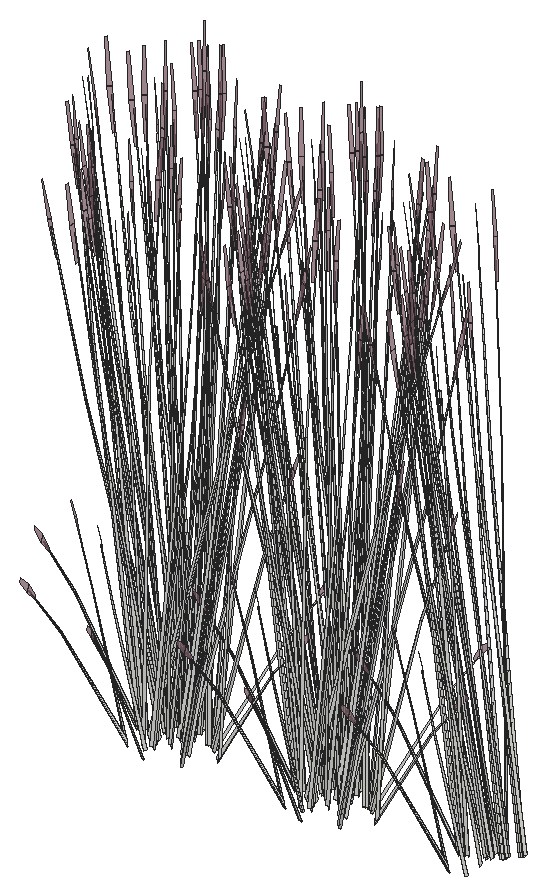
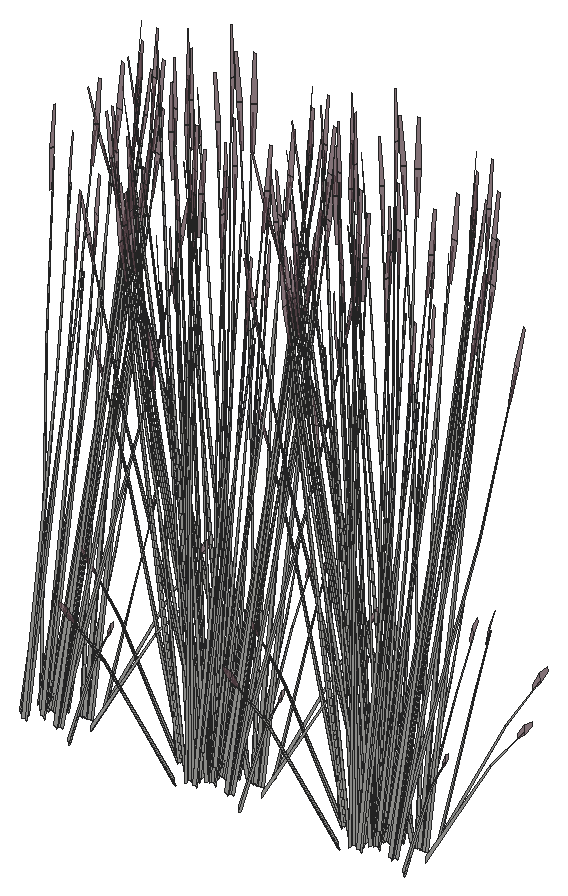
# SketchUp Ruby script. Lengths in inches.
U = 1.inch
M = Sketchup.active_model
def pt(a) = Geom::Point3d.new(a.map { |v| v * U })
def face(e, loops, mat)
  f = e.add_face(loops[0].map { |a| pt(a) })
  loops[1..].each { |l| e.add_face(l.map { |a| pt(a) }).erase! }
  f.material = f.back_material = mat if mat
  f
end
# faces: each face lists its corners as indices into pts; further lists are holes
def faces(e, pts, list, mat = nil) = list.each { |f| face(e, (f[0].is_a?(Array) ? f : [f]).map { |l| l.map { |i| pts[i] } }, mat) }
# xy, xz, yz: faces in a plane at the given z, y or x. An outline is a flat list of corners, or four numbers for a rectangle; further outlines are holes
def ring(l) = l.size == 4 ? [[l[0], l[1]], [l[2], l[1]], [l[2], l[3]], [l[0], l[3]]] : l.each_slice(2).to_a
def flat(e, list, mat, &to3) = list.each { |f| face(e, (f[0].is_a?(Array) ? f : [f]).map { |l| ring(l).map { |u, v| to3.(u, v) } }, mat) }
def xy(e, z, list, mat = nil) = flat(e, list, mat) { |x, y| [x, y, z] }
def xz(e, y, list, mat = nil) = flat(e, list, mat) { |x, z| [x, y, z] }
def yz(e, x, list, mat = nil) = flat(e, list, mat) { |y, z| [x, y, z] }
def lines(e, pts, list) = list.each { |a, b| e.add_line(pt(pts[a]), pt(pts[b])) }
# prism: a flat outline (further loops are holes) pulled along v
def prism(e, loops, v, mat = nil)
  f = face(e, loops, mat); d = Geom::Vector3d.new(v.map { |x| x * U })
  f.pushpull(f.normal.samedirection?(d) ? d.length : -d.length)
end
def box(e, o, s, mat = nil) = prism(e, [[o, [o[0] + s[0], o[1], o[2]], [o[0] + s[0], o[1] + s[1], o[2]], [o[0], o[1] + s[1], o[2]]]], [0, 0, s[2]], mat)
def at(x, y, z, deg = 0) = Geom::Transformation.translation(pt([x, y, z])) * Geom::Transformation.rotation(ORIGIN, Z_AXIS, deg.degrees)
def axes(o, x, y, z) = Geom::Transformation.new([*x, 0, *y, 0, *z, 0, *pt(o).to_a, 1])
def part(name) = M.definitions.add(name)
# library, detail: a bought-in or finely detailed component or shape, given as its bounding box
def library(name, o, s) = part(name).tap { |d| box(d.entities, o, s) }
def detail(e, o, s) = box(e.add_group.entities, o, s)
def put(e, d, t, mat = nil) = e.add_instance(d, t).tap { |i| i.material = mat if mat }
def group(e, t, mat = nil) = e.add_group.tap { |g| g.transformation = t; g.material = mat if mat }.entities
root = M.entities
M.materials.add("LightPink_Translucent").color = [144, 107, 117]
M.materials["LightPink_Translucent"].alpha = 0.75
c1 = part("blade")
p = [[2.15,0.21,22],[0,0.17,0],[0.09,0.45,0],[2.18,0.31,22],[2.29,0.31,22],[0.38,0.45,0],
  [2.48,0.24,33],[2.49,0.24,33],[2.48,0.22,33]]
faces(c1.entities,p,[[0,1,2,3],[4,5,2,3],[6,3,4,7],[8,0,3,6]])
c2 = part("seeds")
p = [[0.3,-0.1,1.38],[-0.01,-0.03,1.59],[-0.01,-0.03,0.03],[0.14,-0.07,-0.07],[0.29,-0.03,3],[0.15,0.01,3.11]]
faces(c2.entities,p,[[0,1,2,3],[1,0,4,5]],"LightPink_Translucent")
c3 = part("blade with seeds")
put(c3.entities,c1,at(0,0,0))
put(c3.entities,c2,axes([2.4,0.25,30.99],[1.5799,-0.05474,1.17369],[-0.12525,1.92788,0.29478],[-0.07173,-0.02425,1.56792]))
put(root,c3,axes([242.16,53.45,256.49],[0.01927,0.0963,1.76342],[-0.38846,0.5029,-0.26939],[-0.27592,-0.02535,0.30037]))
put(root,c3,axes([241.95,56.15,256.49],[0.10192,0.06105,1.76342],[0.17281,0.56562,-0.26939],[-0.22588,0.12062,0.30037]))
put(root,c3,axes([244.7,54.32,257.06],[-0.79037,-0.10018,-0.62353],[0.16679,-0.61794,-0.16365],[-0.23587,-0.07488,1.37633]))
put(root,c3,axes([243.66,55.49,257.02],[-0.7111,-0.30552,-0.49651],[0.42504,-0.54784,0],[-0.16196,-0.06958,1.57504]))
put(root,c3,axes([243.35,50.94,256.49],[-0.0736,0.08049,1.76342],[-0.74378,0.17355,-0.26939],[-0.17968,-0.15788,0.30037]))
put(root,c3,axes([244.1,55.86,257.375],[-0.47504,0.61229,0],[-0.79476,-0.34146,-0.51607],[-0.18101,-0.07777,1.63711]))
put(root,c3,axes([242.89,51.25,257.13],[-0.21918,0.49894,-0.03893],[-0.6746,-0.15348,-0.17649],[-0.10242,-0.08161,0.58215]))
put(root,c3,axes([245.6,54.42,257.67],[-0.76714,0.40567,-0.29095],[-0.51013,-0.57321,-0.50002],[-0.18927,-0.05821,1.59708]))
put(root,c3,axes([242.53,53.53,257.375],[-0.95008,0,0],[0,-0.68292,-0.51607],[0,-0.15554,1.63711]))
put(root,c3,axes([243.86,55.27,257.03],[-0.17848,-0.53243,-0.30978],[0.70886,-0.15119,0.30978],[-0.1429,-0.0614,1.38974]))
put(root,c3,axes([246.11,54.86,257.06],[-0.51177,0.45928,-0.62353],[-0.63575,-0.41646,-0.16365],[-0.20507,0.11457,1.37633]))
put(root,c3,axes([243.26,53.35,257.33],[-0.70674,0.51372,0.30756],[-0.70717,-0.50832,-0.36492],[-0.02468,-0.14589,1.64885]))
put(root,c3,axes([246.46,54.6,257.46],[-0.74193,-0.49181,-0.25192],[0.6243,-0.55226,0.5513],[-0.19979,0.05753,1.68216]))
put(root,c3,axes([245.11,54.13,257.21],[-0.45644,-0.51287,-0.44739],[0.69137,-0.36116,0.21531],[-0.14771,-0.06346,1.43643]))
put(root,c3,axes([246.08,54.5,257.21],[-0.82508,0.03772,-0.44739],[-0.07462,-0.62614,0.21531],[-0.14771,0.06346,1.43643]))
put(root,c3,axes([245.18,54.42,257.4375],[0.20138,-0.72405,-0.23429],[0.95485,0.12621,0.51271],[-0.16685,-0.09999,1.5644]))
put(root,c3,axes([246.95,56.11,257.02],[-0.7111,0.30552,-0.49651],[-0.42504,-0.54784,0],[-0.16196,0.06958,1.57504]))
put(root,c3,axes([242.74,53.07,257.02],[0,-0.61104,-0.49651],[0.85008,0,0],[0,-0.13917,1.57504]))
put(root,c3,axes([247,55.95,257.19],[-0.46912,-0.61443,-0.05142],[0.79476,-0.34146,0.51607],[-0.19584,0.0585,1.6363]))
put(root,c3,axes([246.78,55.87,257.03],[-0.70886,-0.15119,-0.30978],[0.17848,-0.53243,0.30978],[-0.1429,0.0614,1.38974]))
put(root,c3,axes([244.96,53.77,257.67],[-0.85568,-0.29155,-0.29095],[0.41201,-0.61537,-0.50002],[-0.02689,-0.15109,1.59708]))
put(root,c3,axes([246.66,54.33,257.67],[0.08854,0.69723,-0.29095],[-0.92215,0.04216,-0.50002],[-0.16238,0.09287,1.59708]))
put(root,c3,axes([244.58,53.15,257.1],[-0.31203,-0.62659,-0.69835],[0.89884,-0.22566,-0.18329],[-0.03449,-0.21218,1.54149]))
put(root,c3,axes([243.1,53.08,257.03],[0.53038,-0.38124,-0.30978],[0.53038,0.38124,0.30978],[0,-0.1228,1.38974]))
put(root,c3,axes([245.5,50.62,257.13],[-0.52505,0.35054,-0.03893],[-0.48109,-0.38392,-0.17649],[-0.03387,-0.10878,0.58215]))
put(root,c3,axes([245.82,55.33,257.2],[-0.76598,-0.27433,0],[0.36864,-0.57001,0],[0,0,1.62707]))
put(root,c3,axes([247.6,56.02,257.375],[0.47504,0.61229,0],[-0.79476,0.34146,-0.51607],[-0.18101,0.07777,1.63711]))
put(root,c3,axes([246.63,54.01,257.3],[-0.70674,-0.52593,-0.06131],[0.70717,-0.52625,0],[-0.02468,-0.01837,1.75571]))
put(root,c3,axes([247.02,55.63,257.33],[0.95122,0.19861,0.30756],[-0.23797,0.7099,-0.36492],[-0.15744,0.08885,1.64885]))
put(root,c3,axes([245.63,50.1875,256.49],[-0.12744,0.02202,1.76342],[-0.70477,-0.24781,-0.26939],[0.01183,-0.2067,0.30037]))
put(root,c3,axes([245.05,53.32,257.21],[0.36864,-0.55059,-0.44739],[0.76598,0.26498,0.21531],[0,-0.12692,1.43643]))
put(root,c3,axes([246,55.09,257.2],[-0.24791,-0.5268,0],[0.70791,-0.18448,0],[0,0,1.54371]))
put(root,c3,axes([247,54.05,257.21],[-0.36864,0.55059,-0.44739],[-0.76598,-0.26498,0.21531],[0,0.12692,1.43643]))
put(root,c3,axes([246.39,53.46,257.21],[0,-0.70701,0],[0.95008,0,0],[0,0,1.79456]))
put(root,c3,axes([246.87,53.74,257.29],[0,0.70667,-0.05637],[-0.95008,0,0],[0,0.02221,1.79368]))
put(root,c3,axes([246.42,55.11,257.29],[0.33034,0.70197,-0.06012],[-0.94388,0.24598,0],[0.01154,0.02451,1.72173]))
put(root,c3,axes([244.46,51.35,257.375],[-0.47504,-0.61229,0],[0.79476,-0.34146,-0.51607],[0.18101,-0.07777,1.63711]))
put(root,c3,axes([249.14,54.19,257.2],[-0.94962,-0.00489,-0.04976],[0,-0.68292,0.49943],[-0.02984,0.15546,1.58352]))
put(root,c3,axes([247.02,53.89,257.21],[0.53038,0.39469,0],[-0.53038,0.39469,0],[0,0,1.69266]))
put(root,c3,axes([246.69,55.34,257.2],[0.76598,0.27433,0],[-0.36864,0.57001,0],[0,0,1.74954]))
put(root,c3,axes([248.95,54.29,257.03],[-0.53038,0.38124,-0.30978],[-0.53038,-0.38124,0.30978],[0,0.1228,1.38974]))
put(root,c3,axes([247.43,54.22,257.09],[0.2786,0.55945,-0.69212],[-0.80253,0.20149,-0.18165],[0.03079,0.18945,1.52773]))
put(root,c3,axes([247.04,53.62,257.21],[0.85008,0,0],[0,0.63259,0],[0,0,1.78407]))
put(root,c3,axes([245.39,53.04,257.67],[-0.08854,-0.69723,-0.29095],[0.92215,-0.04216,-0.50002],[0.16238,-0.09287,1.59708]))
put(root,c3,axes([247.09,53.6,257.67],[0.85568,0.29155,-0.29095],[-0.41201,0.61537,-0.50002],[0.02689,0.15109,1.59708]))
put(root,c3,axes([245.27,51.5,257.03],[0.70886,0.15119,-0.30978],[-0.17848,0.53243,0.30978],[0.1429,-0.0614,1.38974]))
put(root,c3,axes([249.3125,54.3,257.02],[0,0.61104,-0.49651],[-0.85008,0,0],[0,0.13917,1.57504]))
put(root,c3,axes([245.1,51.26,257.02],[0.7111,-0.30552,-0.49651],[0.42504,0.54784,0],[0.16196,-0.06958,1.57504]))
put(root,c3,axes([246.93,55.02,257.18],[0.79769,-0.20732,-0.19198],[0.2803,0.59721,0.00008],[0.08805,-0.02292,1.73897]))
put(root,c3,axes([246.94,53.24,257.21],[0.45644,0.51287,-0.44739],[-0.69137,0.36116,0.21531],[0.14771,0.06346,1.43643]))
put(root,c3,axes([245.94,52.51,257.06],[0.51177,-0.45928,-0.62353],[0.63575,0.41646,-0.16365],[0.20507,-0.11457,1.37633]))
put(root,c3,axes([248.19,52.1,257.03],[0.17848,0.53243,-0.30978],[-0.70886,0.15119,0.30978],[0.1429,0.0614,1.38974]))
put(root,c3,axes([249.52,53.84,257.375],[0.95008,0,0],[0,0.68292,-0.51607],[0,0.15554,1.63711]))
put(root,c3,axes([246.45,52.95,257.67],[0.76714,-0.40567,-0.29095],[0.51013,0.57321,-0.50002],[0.18927,0.05821,1.59708]))
put(root,c3,axes([244.52,52.59,256.59],[-0.74787,0.24464,1.28929],[-0.23804,-0.70192,0.50096],[0.45924,0.01168,1.46642]))
put(root,c3,axes([247.95,51.51,257.375],[0.47504,-0.61229,0],[0.79476,0.34146,-0.51607],[0.18101,0.07777,1.63711]))
put(root,c3,axes([248.75,51.24,256.49],[-0.11372,-0.04814,1.76342],[-0.29211,-0.53779,-0.26939],[0.19706,-0.14594,0.30037]))
put(root,c3,axes([248.39,51.875,257.02],[0.7111,0.30552,-0.49651],[-0.42504,0.54784,0],[0.16196,0.06958,1.57504]))
put(root,c3,axes([248.35,56.22,256.49],[0.05536,-0.08822,1.76342],[0.69692,-0.25981,-0.26939],[0.21129,0.13447,0.30037]))
put(root,c3,axes([247.35,53.05,257.06],[0.79037,0.10018,-0.62353],[-0.16679,0.61794,-0.16365],[0.23587,0.07488,1.37633]))
put(root,c3,axes([250.72,53.41,257.26],[-0.47106,-0.39072,-0.06488],[0.51591,-0.35801,-0.29416],[0.14618,-0.02521,0.97024]))
put(root,c3,axes([258.23,53.45,256.49],[0.01927,0.0963,1.76342],[-0.38846,0.5029,-0.26939],[-0.27592,-0.02535,0.30037]))
put(root,c3,axes([258.02,56.15,256.49],[0.10192,0.06105,1.76342],[0.17281,0.56562,-0.26939],[-0.22588,0.12062,0.30037]))
put(root,c3,axes([249.82,53.93,256.98],[-0.48937,0.07333,1.41583],[-0.07789,-0.58369,0.08104],[0.34275,-0.08835,0.80566]))
put(root,c3,axes([250.36,53.55,256.49],[-0.03971,-0.09277,1.76342],[0.27541,-0.54264,-0.26939],[0.27782,-0.00781,0.30037]))
put(root,c3,axes([260.77,54.32,257.06],[-0.79037,-0.10018,-0.62353],[0.16679,-0.61794,-0.16365],[-0.23587,-0.07488,1.37633]))
put(root,c3,axes([259.73,55.49,257.02],[-0.7111,-0.30552,-0.49651],[0.42504,-0.54784,0],[-0.16196,-0.06958,1.57504]))
put(root,c3,axes([259.42,50.94,256.49],[-0.0736,0.08049,1.76342],[-0.74378,0.17355,-0.26939],[-0.17968,-0.15788,0.30037]))
put(root,c3,axes([260.16,55.86,257.375],[-0.47504,0.61229,0],[-0.79476,-0.34146,-0.51607],[-0.18101,-0.07777,1.63711]))
put(root,c3,axes([258.95,51.25,257.13],[-0.21918,0.49894,-0.03893],[-0.6746,-0.15348,-0.17649],[-0.10242,-0.08161,0.58215]))
put(root,c3,axes([261.66,54.42,257.67],[-0.76714,0.40567,-0.29095],[-0.51013,-0.57321,-0.50002],[-0.18927,-0.05821,1.59708]))
put(root,c3,axes([258.59,53.53,257.375],[-0.95008,0,0],[0,-0.68292,-0.51607],[0,-0.15554,1.63711]))
put(root,c3,axes([259.93,55.27,257.03],[-0.17848,-0.53243,-0.30978],[0.70886,-0.15119,0.30978],[-0.1429,-0.0614,1.38974]))
put(root,c3,axes([262.17,54.86,257.06],[-0.51177,0.45928,-0.62353],[-0.63575,-0.41646,-0.16365],[-0.20507,0.11457,1.37633]))
put(root,c3,axes([259.33,53.35,257.33],[-0.70674,0.51372,0.30756],[-0.70717,-0.50832,-0.36492],[-0.02468,-0.14589,1.64885]))
put(root,c3,axes([262.52,54.6,257.46],[-0.74193,-0.49181,-0.25192],[0.6243,-0.55226,0.5513],[-0.19979,0.05753,1.68216]))
put(root,c3,axes([261.18,54.13,257.21],[-0.45644,-0.51287,-0.44739],[0.69137,-0.36116,0.21531],[-0.14771,-0.06346,1.43643]))
put(root,c3,axes([262.15,54.5,257.21],[-0.82508,0.03772,-0.44739],[-0.07462,-0.62614,0.21531],[-0.14771,0.06346,1.43643]))
put(root,c3,axes([261.24,54.42,257.4375],[0.20138,-0.72405,-0.23429],[0.95485,0.12621,0.51271],[-0.16685,-0.09999,1.5644]))
put(root,c3,axes([263.02,56.11,257.02],[-0.7111,0.30552,-0.49651],[-0.42504,-0.54784,0],[-0.16196,0.06958,1.57504]))
put(root,c3,axes([258.81,53.07,257.02],[0,-0.61104,-0.49651],[0.85008,0,0],[0,-0.13917,1.57504]))
put(root,c3,axes([263.0625,55.95,257.19],[-0.46912,-0.61443,-0.05142],[0.79476,-0.34146,0.51607],[-0.19584,0.0585,1.6363]))
put(root,c3,axes([262.85,55.87,257.03],[-0.70886,-0.15119,-0.30978],[0.17848,-0.53243,0.30978],[-0.1429,0.0614,1.38974]))
put(root,c3,axes([261.03,53.77,257.67],[-0.85568,-0.29155,-0.29095],[0.41201,-0.61537,-0.50002],[-0.02689,-0.15109,1.59708]))
put(root,c3,axes([262.73,54.33,257.67],[0.08854,0.69723,-0.29095],[-0.92215,0.04216,-0.50002],[-0.16238,0.09287,1.59708]))
put(root,c3,axes([260.64,53.15,257.1],[-0.31203,-0.62659,-0.69835],[0.89884,-0.22566,-0.18329],[-0.03449,-0.21218,1.54149]))
put(root,c3,axes([259.17,53.08,257.03],[0.53038,-0.38124,-0.30978],[0.53038,0.38124,0.30978],[0,-0.1228,1.38974]))
put(root,c3,axes([261.56,50.62,257.13],[-0.52505,0.35054,-0.03893],[-0.48109,-0.38392,-0.17649],[-0.03387,-0.10878,0.58215]))
put(root,c3,axes([261.89,55.33,257.2],[-0.76598,-0.27433,0],[0.36864,-0.57001,0],[0,0,1.62707]))
put(root,c3,axes([263.66,56.02,257.375],[0.47504,0.61229,0],[-0.79476,0.34146,-0.51607],[-0.18101,0.07777,1.63711]))
put(root,c3,axes([262.7,54.01,257.3],[-0.70674,-0.52593,-0.06131],[0.70717,-0.52625,0],[-0.02468,-0.01837,1.75571]))
put(root,c3,axes([263.08,55.63,257.33],[0.95122,0.19861,0.30756],[-0.23797,0.7099,-0.36492],[-0.15744,0.08885,1.64885]))
put(root,c3,axes([261.7,50.1875,256.49],[-0.12744,0.02202,1.76342],[-0.70477,-0.24781,-0.26939],[0.01183,-0.2067,0.30037]))
put(root,c3,axes([261.12,53.32,257.21],[0.36864,-0.55059,-0.44739],[0.76598,0.26498,0.21531],[0,-0.12692,1.43643]))
put(root,c3,axes([262.0625,55.09,257.2],[-0.24791,-0.5268,0],[0.70791,-0.18448,0],[0,0,1.54371]))
put(root,c3,axes([263.0625,54.05,257.21],[-0.36864,0.55059,-0.44739],[-0.76598,-0.26498,0.21531],[0,0.12692,1.43643]))
put(root,c3,axes([262.46,53.46,257.21],[0,-0.70701,0],[0.95008,0,0],[0,0,1.79456]))
put(root,c3,axes([262.9375,53.74,257.29],[0,0.70667,-0.05637],[-0.95008,0,0],[0,0.02221,1.79368]))
put(root,c3,axes([262.48,55.11,257.29],[0.33034,0.70197,-0.06012],[-0.94388,0.24598,0],[0.01154,0.02451,1.72173]))
put(root,c3,axes([260.52,51.35,257.375],[-0.47504,-0.61229,0],[0.79476,-0.34146,-0.51607],[0.18101,-0.07777,1.63711]))
put(root,c3,axes([265.21,54.19,257.2],[-0.94962,-0.00489,-0.04976],[0,-0.68292,0.49943],[-0.02984,0.15546,1.58352]))
put(root,c3,axes([263.08,53.89,257.21],[0.53038,0.39469,0],[-0.53038,0.39469,0],[0,0,1.69266]))
put(root,c3,axes([262.76,55.34,257.2],[0.76598,0.27433,0],[-0.36864,0.57001,0],[0,0,1.74954]))
put(root,c3,axes([265.01,54.29,257.03],[-0.53038,0.38124,-0.30978],[-0.53038,-0.38124,0.30978],[0,0.1228,1.38974]))
put(root,c3,axes([263.5,54.22,257.09],[0.2786,0.55945,-0.69212],[-0.80253,0.20149,-0.18165],[0.03079,0.18945,1.52773]))
put(root,c3,axes([263.1,53.62,257.21],[0.85008,0,0],[0,0.63259,0],[0,0,1.78407]))
put(root,c3,axes([261.46,53.04,257.67],[-0.08854,-0.69723,-0.29095],[0.92215,-0.04216,-0.50002],[0.16238,-0.09287,1.59708]))
put(root,c3,axes([263.16,53.6,257.67],[0.85568,0.29155,-0.29095],[-0.41201,0.61537,-0.50002],[0.02689,0.15109,1.59708]))
put(root,c3,axes([261.33,51.5,257.03],[0.70886,0.15119,-0.30978],[-0.17848,0.53243,0.30978],[0.1429,-0.0614,1.38974]))
put(root,c3,axes([265.38,54.3,257.02],[0,0.61104,-0.49651],[-0.85008,0,0],[0,0.13917,1.57504]))
put(root,c3,axes([261.17,51.26,257.02],[0.7111,-0.30552,-0.49651],[0.42504,0.54784,0],[0.16196,-0.06958,1.57504]))
put(root,c3,axes([262.99,55.02,257.18],[0.79769,-0.20732,-0.19198],[0.2803,0.59721,0.00008],[0.08805,-0.02292,1.73897]))
put(root,c3,axes([263.01,53.24,257.21],[0.45644,0.51287,-0.44739],[-0.69137,0.36116,0.21531],[0.14771,0.06346,1.43643]))
put(root,c3,axes([262.01,52.51,257.06],[0.51177,-0.45928,-0.62353],[0.63575,0.41646,-0.16365],[0.20507,-0.11457,1.37633]))
put(root,c3,axes([264.26,52.1,257.03],[0.17848,0.53243,-0.30978],[-0.70886,0.15119,0.30978],[0.1429,0.0614,1.38974]))
put(root,c3,axes([265.59,53.84,257.375],[0.95008,0,0],[0,0.68292,-0.51607],[0,0.15554,1.63711]))
put(root,c3,axes([262.52,52.95,257.67],[0.76714,-0.40567,-0.29095],[0.51013,0.57321,-0.50002],[0.18927,0.05821,1.59708]))
put(root,c3,axes([260.58,52.59,256.59],[-0.74787,0.24464,1.28929],[-0.23804,-0.70192,0.50096],[0.45924,0.01168,1.46642]))
put(root,c3,axes([264.02,51.51,257.375],[0.47504,-0.61229,0],[0.79476,0.34146,-0.51607],[0.18101,0.07777,1.63711]))
put(root,c3,axes([264.82,51.24,256.49],[-0.11372,-0.04814,1.76342],[-0.29211,-0.53779,-0.26939],[0.19706,-0.14594,0.30037]))
put(root,c3,axes([264.45,51.875,257.02],[0.7111,0.30552,-0.49651],[-0.42504,0.54784,0],[0.16196,0.06958,1.57504]))
put(root,c3,axes([264.42,56.22,256.49],[0.05536,-0.08822,1.76342],[0.69692,-0.25981,-0.26939],[0.21129,0.13447,0.30037]))
put(root,c3,axes([263.42,53.05,257.06],[0.79037,0.10018,-0.62353],[-0.16679,0.61794,-0.16365],[0.23587,0.07488,1.37633]))
put(root,c3,axes([266.78,53.41,257.26],[-0.47106,-0.39072,-0.06488],[0.51591,-0.35801,-0.29416],[0.14618,-0.02521,0.97024]))
put(root,c3,axes([274.95,53.45,256.49],[0.01927,0.0963,1.76342],[-0.38846,0.5029,-0.26939],[-0.27592,-0.02535,0.30037]))
put(root,c3,axes([274.75,56.15,256.49],[0.10192,0.06105,1.76342],[0.17281,0.56562,-0.26939],[-0.22588,0.12062,0.30037]))
put(root,c3,axes([265.89,53.93,256.98],[-0.48937,0.07333,1.41583],[-0.07789,-0.58369,0.08104],[0.34275,-0.08835,0.80566]))
put(root,c3,axes([266.42,53.55,256.49],[-0.03971,-0.09277,1.76342],[0.27541,-0.54264,-0.26939],[0.27782,-0.00781,0.30037]))
put(root,c3,axes([277.49,54.32,257.06],[-0.79037,-0.10018,-0.62353],[0.16679,-0.61794,-0.16365],[-0.23587,-0.07488,1.37633]))
put(root,c3,axes([276.46,55.49,257.02],[-0.7111,-0.30552,-0.49651],[0.42504,-0.54784,0],[-0.16196,-0.06958,1.57504]))
put(root,c3,axes([276.15,50.94,256.49],[-0.0736,0.08049,1.76342],[-0.74378,0.17355,-0.26939],[-0.17968,-0.15788,0.30037]))
put(root,c3,axes([276.89,55.86,257.375],[-0.47504,0.61229,0],[-0.79476,-0.34146,-0.51607],[-0.18101,-0.07777,1.63711]))
put(root,c3,axes([275.68,51.25,257.13],[-0.21918,0.49894,-0.03893],[-0.6746,-0.15348,-0.17649],[-0.10242,-0.08161,0.58215]))
put(root,c3,axes([278.39,54.42,257.67],[-0.76714,0.40567,-0.29095],[-0.51013,-0.57321,-0.50002],[-0.18927,-0.05821,1.59708]))
put(root,c3,axes([275.32,53.53,257.375],[-0.95008,0,0],[0,-0.68292,-0.51607],[0,-0.15554,1.63711]))
put(root,c3,axes([276.66,55.27,257.03],[-0.17848,-0.53243,-0.30978],[0.70886,-0.15119,0.30978],[-0.1429,-0.0614,1.38974]))
put(root,c3,axes([278.9,54.86,257.06],[-0.51177,0.45928,-0.62353],[-0.63575,-0.41646,-0.16365],[-0.20507,0.11457,1.37633]))
put(root,c3,axes([276.06,53.35,257.33],[-0.70674,0.51372,0.30756],[-0.70717,-0.50832,-0.36492],[-0.02468,-0.14589,1.64885]))
put(root,c3,axes([279.25,54.6,257.46],[-0.74193,-0.49181,-0.25192],[0.6243,-0.55226,0.5513],[-0.19979,0.05753,1.68216]))
put(root,c3,axes([277.9,54.13,257.21],[-0.45644,-0.51287,-0.44739],[0.69137,-0.36116,0.21531],[-0.14771,-0.06346,1.43643]))
put(root,c3,axes([278.875,54.5,257.21],[-0.82508,0.03772,-0.44739],[-0.07462,-0.62614,0.21531],[-0.14771,0.06346,1.43643]))
put(root,c3,axes([277.97,54.42,257.4375],[0.20138,-0.72405,-0.23429],[0.95485,0.12621,0.51271],[-0.16685,-0.09999,1.5644]))
put(root,c3,axes([279.74,56.11,257.02],[-0.7111,0.30552,-0.49651],[-0.42504,-0.54784,0],[-0.16196,0.06958,1.57504]))
put(root,c3,axes([275.53,53.07,257.02],[0,-0.61104,-0.49651],[0.85008,0,0],[0,-0.13917,1.57504]))
put(root,c3,axes([279.79,55.95,257.19],[-0.46912,-0.61443,-0.05142],[0.79476,-0.34146,0.51607],[-0.19584,0.0585,1.6363]))
put(root,c3,axes([279.58,55.87,257.03],[-0.70886,-0.15119,-0.30978],[0.17848,-0.53243,0.30978],[-0.1429,0.0614,1.38974]))
put(root,c3,axes([277.76,53.77,257.67],[-0.85568,-0.29155,-0.29095],[0.41201,-0.61537,-0.50002],[-0.02689,-0.15109,1.59708]))
put(root,c3,axes([279.46,54.33,257.67],[0.08854,0.69723,-0.29095],[-0.92215,0.04216,-0.50002],[-0.16238,0.09287,1.59708]))
put(root,c3,axes([277.37,53.15,257.1],[-0.31203,-0.62659,-0.69835],[0.89884,-0.22566,-0.18329],[-0.03449,-0.21218,1.54149]))
put(root,c3,axes([275.9,53.08,257.03],[0.53038,-0.38124,-0.30978],[0.53038,0.38124,0.30978],[0,-0.1228,1.38974]))
put(root,c3,axes([278.29,50.62,257.13],[-0.52505,0.35054,-0.03893],[-0.48109,-0.38392,-0.17649],[-0.03387,-0.10878,0.58215]))
